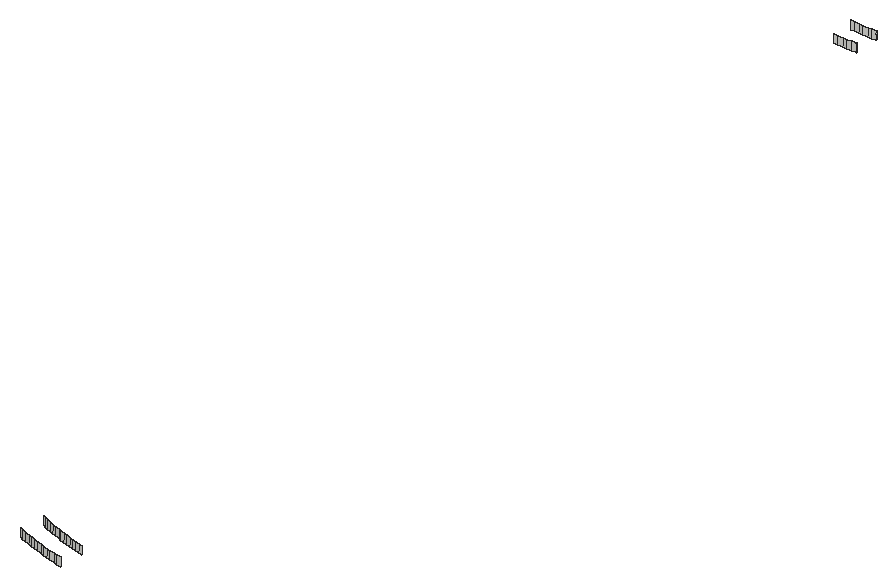
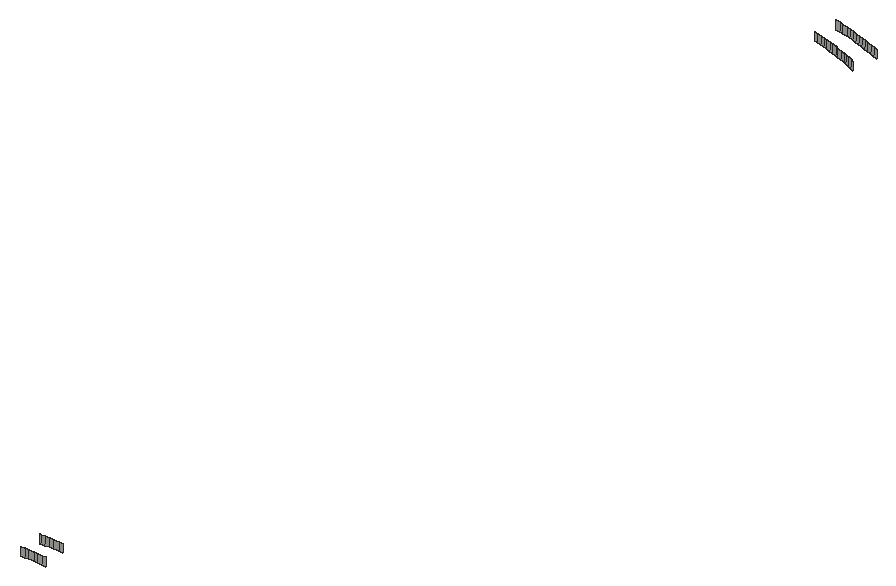
# SketchUp Ruby script. Lengths in inches.
U = 1.inch
M = Sketchup.active_model
def pt(a) = Geom::Point3d.new(a.map { |v| v * U })
def face(e, loops, mat)
  f = e.add_face(loops[0].map { |a| pt(a) })
  loops[1..].each { |l| e.add_face(l.map { |a| pt(a) }).erase! }
  f.material = f.back_material = mat if mat
  f
end
# faces: each face lists its corners as indices into pts; further lists are holes
def faces(e, pts, list, mat = nil) = list.each { |f| face(e, (f[0].is_a?(Array) ? f : [f]).map { |l| l.map { |i| pts[i] } }, mat) }
# xy, xz, yz: faces in a plane at the given z, y or x. An outline is a flat list of corners, or four numbers for a rectangle; further outlines are holes
def ring(l) = l.size == 4 ? [[l[0], l[1]], [l[2], l[1]], [l[2], l[3]], [l[0], l[3]]] : l.each_slice(2).to_a
def flat(e, list, mat, &to3) = list.each { |f| face(e, (f[0].is_a?(Array) ? f : [f]).map { |l| ring(l).map { |u, v| to3.(u, v) } }, mat) }
def xy(e, z, list, mat = nil) = flat(e, list, mat) { |x, y| [x, y, z] }
def xz(e, y, list, mat = nil) = flat(e, list, mat) { |x, z| [x, y, z] }
def yz(e, x, list, mat = nil) = flat(e, list, mat) { |y, z| [x, y, z] }
def lines(e, pts, list) = list.each { |a, b| e.add_line(pt(pts[a]), pt(pts[b])) }
# prism: a flat outline (further loops are holes) pulled along v
def prism(e, loops, v, mat = nil)
  f = face(e, loops, mat); d = Geom::Vector3d.new(v.map { |x| x * U })
  f.pushpull(f.normal.samedirection?(d) ? d.length : -d.length)
end
def box(e, o, s, mat = nil) = prism(e, [[o, [o[0] + s[0], o[1], o[2]], [o[0] + s[0], o[1] + s[1], o[2]], [o[0], o[1] + s[1], o[2]]]], [0, 0, s[2]], mat)
def at(x, y, z, deg = 0) = Geom::Transformation.translation(pt([x, y, z])) * Geom::Transformation.rotation(ORIGIN, Z_AXIS, deg.degrees)
def axes(o, x, y, z) = Geom::Transformation.new([*x, 0, *y, 0, *z, 0, *pt(o).to_a, 1])
def part(name) = M.definitions.add(name)
# library, detail: a bought-in or finely detailed component or shape, given as its bounding box
def library(name, o, s) = part(name).tap { |d| box(d.entities, o, s) }
def detail(e, o, s) = box(e.add_group.entities, o, s)
def put(e, d, t, mat = nil) = e.add_instance(d, t).tap { |i| i.material = mat if mat }
def group(e, t, mat = nil) = e.add_group.tap { |g| g.transformation = t; g.material = mat if mat }.entities
root = M.entities
xz(root,186.5,[[151.71,116,151.95,116.5],[151.95,116,152,116.5]])
xz(root,188,[[151.73,116,151.96,116.5],[151.96,116,152,116.5]])
xz(root,188.01,[[151.2,116,151.47,116.5]])
p = [[153.59,124.49,116],[153.33,124.55,116],[153.33,124.55,116.5],[153.59,124.49,116.5],[153.08,124.62,116],[152.82,124.68,116],
  [152.82,124.68,116.5],[153.08,124.62,116.5],[152.57,124.75,116],[152.57,124.75,116.5],[152.32,124.82,116],[152.07,124.9,116],
  [152.07,124.9,116.5],[152.32,124.82,116.5],[151.82,124.98,116],[151.82,124.98,116.5],[151.57,125.0625,116],[151.57,125.0625,116.5],
  [151.32,125.15,116],[151.08,125.24,116],[151.08,125.24,116.5],[151.32,125.15,116.5],[150.83,125.33,116],[150.83,125.33,116.5],
  [150.59,125.42,116],[150.59,125.42,116.5],[150.35,125.52,116],[150.35,125.52,116.5],[153.45,126.07,116],[153.68,126.01,116],
  [153.68,126.01,116.5],[153.45,126.07,116.5],[152.98,126.19,116],[153.21,126.13,116],[153.21,126.13,116.5],[152.98,126.19,116.5],
  [152.75,126.26,116],[152.75,126.26,116.5],[152.28,126.41,116],[152.51,126.33,116],[152.51,126.33,116.5],[152.28,126.41,116.5],
  [152.05,126.48,116],[152.05,126.48,116.5],[151.82,126.5625,116],[151.82,126.5625,116.5],[151.37,126.73,116],[151.6,126.64,116],
  [151.6,126.64,116.5],[151.37,126.73,116.5],[151.14,126.82,116],[151.14,126.82,116.5],[150.92,126.91,116],[150.92,126.91,116.5],
  [150.7,127,116],[150.7,127,116.5],[150.48,127.1,116],[150.48,127.1,116.5],[150.86,186.53,116],[150.58,186.54,116],
  [150.58,186.54,116.5],[150.86,186.53,116.5],[151.15,186.52,116],[151.15,186.52,116.5],[151.43,186.51,116],[151.43,186.51,116.5],
  [151.71,186.5,116],[151.71,186.5,116.5],[150.41,188.06,116],[150.67,188.04,116],[150.67,188.04,116.5],[150.41,188.06,116.5],
  [150.9375,188.03,116],[150.9375,188.03,116.5],[151.2,188.01,116],[151.2,188.01,116.5],[151.47,188.01,116],[151.73,188,116],
  [151.73,188,116.5],[151.47,188.01,116.5]]
faces(root,p,[[0,1,2,3],[4,5,6,7],[1,4,7,2],[5,8,9,6],[10,11,12,13],[8,10,13,9],[11,14,15,12],[14,16,17,15],
  [18,19,20,21],[16,18,21,17],[19,22,23,20],[22,24,25,23],[24,26,27,25],[28,29,30,31],[32,33,34,35],[33,28,31,34],
  [36,32,35,37],[38,39,40,41],[39,36,37,40],[42,38,41,43],[44,42,43,45],[46,47,48,49],[47,44,45,48],[50,46,49,51],
  [52,50,51,53],[54,52,53,55],[56,54,55,57],[58,59,60,61],[62,58,61,63],[64,62,63,65],[66,64,65,67],[68,69,70,71],
  [69,72,73,70],[72,74,75,73],[76,77,78,79]])
